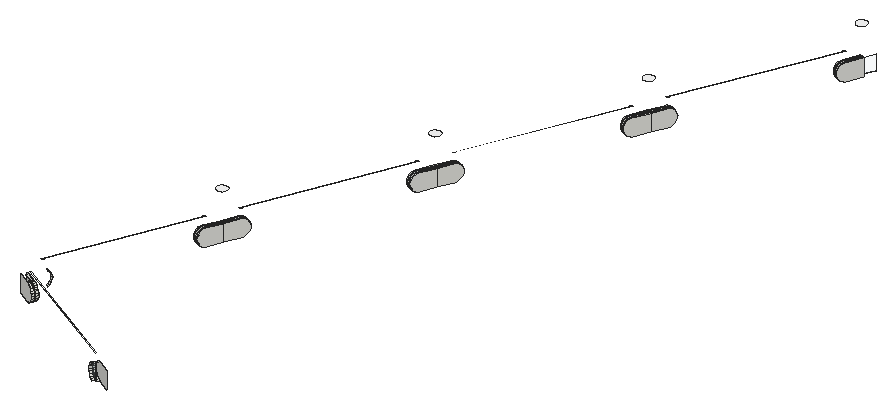
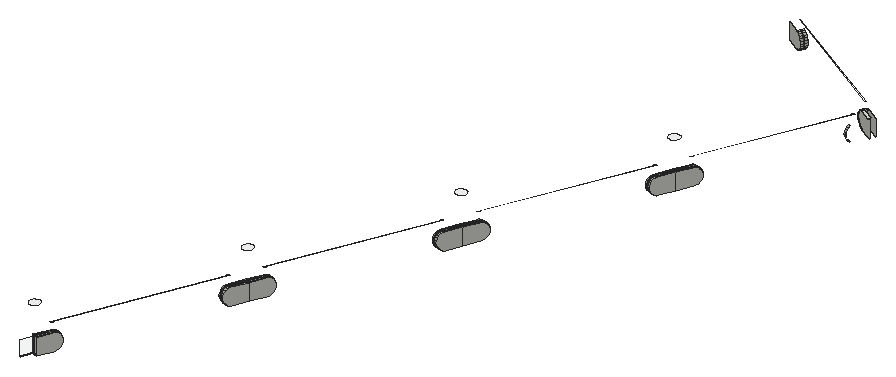
# SketchUp Ruby script. Lengths in inches.
U = 1.inch
M = Sketchup.active_model
def pt(a) = Geom::Point3d.new(a.map { |v| v * U })
def face(e, loops, mat)
  f = e.add_face(loops[0].map { |a| pt(a) })
  loops[1..].each { |l| e.add_face(l.map { |a| pt(a) }).erase! }
  f.material = f.back_material = mat if mat
  f
end
# faces: each face lists its corners as indices into pts; further lists are holes
def faces(e, pts, list, mat = nil) = list.each { |f| face(e, (f[0].is_a?(Array) ? f : [f]).map { |l| l.map { |i| pts[i] } }, mat) }
# xy, xz, yz: faces in a plane at the given z, y or x. An outline is a flat list of corners, or four numbers for a rectangle; further outlines are holes
def ring(l) = l.size == 4 ? [[l[0], l[1]], [l[2], l[1]], [l[2], l[3]], [l[0], l[3]]] : l.each_slice(2).to_a
def flat(e, list, mat, &to3) = list.each { |f| face(e, (f[0].is_a?(Array) ? f : [f]).map { |l| ring(l).map { |u, v| to3.(u, v) } }, mat) }
def xy(e, z, list, mat = nil) = flat(e, list, mat) { |x, y| [x, y, z] }
def xz(e, y, list, mat = nil) = flat(e, list, mat) { |x, z| [x, y, z] }
def yz(e, x, list, mat = nil) = flat(e, list, mat) { |y, z| [x, y, z] }
def lines(e, pts, list) = list.each { |a, b| e.add_line(pt(pts[a]), pt(pts[b])) }
# prism: a flat outline (further loops are holes) pulled along v
def prism(e, loops, v, mat = nil)
  f = face(e, loops, mat); d = Geom::Vector3d.new(v.map { |x| x * U })
  f.pushpull(f.normal.samedirection?(d) ? d.length : -d.length)
end
def box(e, o, s, mat = nil) = prism(e, [[o, [o[0] + s[0], o[1], o[2]], [o[0] + s[0], o[1] + s[1], o[2]], [o[0], o[1] + s[1], o[2]]]], [0, 0, s[2]], mat)
def at(x, y, z, deg = 0) = Geom::Transformation.translation(pt([x, y, z])) * Geom::Transformation.rotation(ORIGIN, Z_AXIS, deg.degrees)
def axes(o, x, y, z) = Geom::Transformation.new([*x, 0, *y, 0, *z, 0, *pt(o).to_a, 1])
def part(name) = M.definitions.add(name)
# library, detail: a bought-in or finely detailed component or shape, given as its bounding box
def library(name, o, s) = part(name).tap { |d| box(d.entities, o, s) }
def detail(e, o, s) = box(e.add_group.entities, o, s)
def put(e, d, t, mat = nil) = e.add_instance(d, t).tap { |i| i.material = mat if mat }
def group(e, t, mat = nil) = e.add_group.tap { |g| g.transformation = t; g.material = mat if mat }.entities
root = M.entities
M.materials.add("Glass_Safety_01").color = [204, 235, 244]
M.materials["Glass_Safety_01"].alpha = 0.1
M.materials.add("[Color_000]").color = [255, 255, 255]
xy(root,351.28,[[970.32,886.89,970.06,887,970.13,887.16,970.85,888.81,971.1,888.7],[969.88,887.08,969.63,887.1875,970.42,888.99,970.67,888.88,969.95,887.24],[971.1,888.7,970.85,888.81,971.64,890.61,971.89,890.5],[970.67,888.88,970.42,888.99,971.2,890.8,971.46,890.6875],[979.95,909,979.69,909.11,979.76,909.25,980.48,910.91,980.73,910.8],
  [979.51,909.1875,979.26,909.3,980.05,911.1,980.3,910.99,979.58,909.33],[980.73,910.8,980.48,910.91,981.27,912.72,981.52,912.61],[980.3,910.99,980.05,911.1,980.83,912.91,981.08,912.8],[989.59,931.14,989.34,931.25,989.4,931.39,990.12,933.05,990.375,932.94],[989.16,931.33,988.9,931.4375,989.6875,933.24,989.94,933.13,989.22,931.47],
  [990.375,932.94,990.12,933.05,990.91,934.86,991.16,934.75],[989.94,933.13,989.6875,933.24,990.47,935.05,990.73,934.9375],[999.21,953.22,998.95,953.33,999.02,953.48,999.74,955.13,999.99,955.02],[998.77,953.41,998.52,953.52,999.31,955.32,999.56,955.21,998.84,953.56]])
xy(root,351.36,[[970.22,887.36,970.04,887.44,970.67,888.88,970.85,888.81],[970.85,888.81,970.67,888.88,971.3,890.33,971.48,890.25],[979.85,909.47,979.67,909.55,980.3,910.99,980.48,910.91],[980.48,910.91,980.3,910.99,980.93,912.43,981.11,912.36],[989.49,931.61,989.3125,931.6875,989.94,933.13,990.12,933.05],
  [990.12,933.05,989.94,933.13,990.57,934.57,990.75,934.5],[999.11,953.69,998.93,953.77,999.56,955.21,999.74,955.13],[999.74,955.13,999.56,955.21,1000.1875,956.66,1000.37,956.58]],"Glass_Safety_01")
xy(root,353.33,[[970.22,887.36,970.85,888.81,970.67,888.88,970.04,887.44],[970.85,888.81,971.48,890.25,971.3,890.33,970.67,888.88],[979.85,909.47,980.48,910.91,980.3,910.99,979.67,909.55],[980.48,910.91,981.11,912.36,980.93,912.43,980.3,910.99],[989.49,931.61,990.12,933.05,989.94,933.13,989.3125,931.6875],
  [990.12,933.05,990.75,934.5,990.57,934.57,989.94,933.13],[999.11,953.69,999.74,955.13,999.56,955.21,998.93,953.77]],"Glass_Safety_01")
xy(root,353.41,[[963.5625,867.39,963.7,867.63,962.28,868.4375,962.17,868.18,963.41,867.48],[970.32,886.89,971.1,888.7,970.85,888.81,970.13,887.16,970.06,887],[969.88,887.08,969.95,887.24,970.67,888.88,970.42,888.99,969.63,887.1875],[971.1,888.7,971.89,890.5,971.64,890.61,970.85,888.81],[970.67,888.88,971.46,890.6875,971.2,890.8,970.42,888.99],
  [979.95,909,980.73,910.8,980.48,910.91,979.76,909.25,979.69,909.11],[979.51,909.1875,979.58,909.33,980.3,910.99,980.05,911.1,979.26,909.3],[980.73,910.8,981.52,912.61,981.27,912.72,980.48,910.91],[980.3,910.99,981.08,912.8,980.83,912.91,980.05,911.1],[989.59,931.14,990.375,932.94,990.12,933.05,989.4,931.39,989.34,931.25],
  [989.16,931.33,989.22,931.47,989.94,933.13,989.6875,933.24,988.9,931.4375],[990.375,932.94,991.16,934.75,990.91,934.86,990.12,933.05],[989.94,933.13,990.73,934.9375,990.47,935.05,989.6875,933.24],[999.21,953.22,999.99,955.02,999.74,955.13,999.02,953.48,998.95,953.33],[998.77,953.41,998.84,953.56,999.56,955.21,999.31,955.32,998.52,953.52]])
xy(root,354.51,[[978.84,858.44,978.9375,858.62,963.31,867.31],[978.9375,858.62,963.41,867.48,963.31,867.31],[962.68,870.04,969.95,887.24,962.5,870.12],[962.68,870.04,970.13,887.16,969.95,887.24],[971.64,890.61,979.58,909.33,971.46,890.6875],
  [971.64,890.61,979.76,909.25,979.58,909.33],[981.27,912.72,989.22,931.47,981.08,912.8],[981.27,912.72,989.4,931.39,989.22,931.47],[990.91,934.86,998.84,953.56,990.73,934.9375],[990.91,934.86,999.02,953.48,998.84,953.56]],"Glass_Safety_01")
xy(root,357.27,[[970.81,888.22,970.97,888.25,971.11,888.32,971.24,888.43,971.33,888.57,971.38,888.73,971.39,888.89,971.36,889.05,971.28,889.2,971.17,889.32,971.04,889.41,970.88,889.46,970.72,889.47,970.55,889.44,970.41,889.37,970.28,889.26,970.19,889.12,970.14,888.96,970.13,888.8,970.17,888.64,970.24,888.49,970.35,888.37,970.49,888.28,970.64,888.23],[980.43,910.32,980.6,910.36,980.74,910.43,980.87,910.54,980.96,910.68,981.01,910.83,981.02,911,980.98,911.16,980.91,911.3,980.8,911.43,980.66,911.52,980.51,911.57,980.34,911.58,980.18,911.55,980.04,911.47,979.91,911.36,979.82,911.23,979.77,911.07,979.76,910.91,979.79,910.75,979.87,910.6,979.98,910.48,980.11,910.39,980.27,910.33],[990.08,932.46,990.24,932.5,990.38,932.57,990.51,932.68,990.6,932.82,990.65,932.97,990.66,933.14,990.625,933.3,990.55,933.44,990.44,933.57,990.31,933.66,990.15,933.71,989.99,933.72,989.83,933.6875,989.68,933.61,989.56,933.5,989.46,933.37,989.41,933.21,989.4,933.05,989.4375,932.89,989.51,932.74,989.62,932.62,989.76,932.53,989.91,932.47],[999.69,954.54,999.85,954.58,1000,954.65,1000.125,954.76,1000.22,954.9,1000.27,955.05,1000.28,955.22,1000.24,955.38,1000.17,955.53,1000.0625,955.65,999.92,955.74,999.77,955.79,999.6,955.8,999.44,955.77,999.3,955.69,999.17,955.59,999.08,955.45,999.03,955.29,999.02,955.13,999.05,954.97,999.13,954.82,999.24,954.7,999.375,954.61,999.53,954.55]],"[Color_000]")
p = [[980.72,857.91,353.41],[980.78,857.88,353.41],[980.78,857.88,351.28],[980.72,857.91,351.28],[979.07,858.85,351.28],[978.83,858.99,351.32],
  [978.61,859.12,351.43],[978.42,859.23,351.59],[978.27,859.3125,351.8125],[978.18,859.36,352.07],[978.15,859.38,352.35],[978.18,859.36,352.62],
  [978.27,859.3125,352.88],[978.42,859.23,353.1],[978.61,859.12,353.27],[978.83,858.99,353.37],[979.07,858.85,353.41],[978.375,858.71,351.43],
  [978.6,858.58,351.32],[978.46,858.34,351.32],[978.24,858.47,351.43],[978.84,858.44,351.28],[978.84,858.44,353.41],[978.6,858.58,353.37],
  [978.375,858.71,353.27],[978.1875,858.82,353.1],[978.04,858.9,352.88],[977.95,858.95,352.62],[977.92,858.97,352.35],[977.95,858.95,352.07],
  [978.04,858.9,351.8125],[978.1875,858.82,351.59],[978.9375,858.62,353.41],[978.9375,858.62,351.28],[978.7,858.75,351.32],[978.47,858.88,351.43],
  [978.28,858.99,351.59],[978.14,859.07,351.8125],[978.04,859.125,352.07],[978.01,859.14,352.35],[978.04,859.125,352.62],[978.14,859.07,352.88],
  [978.28,858.99,353.1],[978.47,858.88,353.27],[978.7,858.75,353.37],[963.33,866.98,353.41],[961.62,867.95,353.41],[961.62,867.95,351.28],
  [963.33,866.98,351.28],[963.57,866.84,351.32],[963.79,866.71,351.43],[963.98,866.61,351.59],[964.13,866.52,351.8125],[964.22,866.47,352.07],
  [964.25,866.45,352.35],[964.22,866.47,352.62],[964.13,866.52,352.88],[963.98,866.61,353.1],[963.79,866.71,353.27],[963.57,866.84,353.37],
  [963.46,867.22,351.28],[963.31,867.31,351.28],[963.31,867.31,353.41],[963.46,867.22,353.41],[963.7,867.08,353.37],[963.93,866.95,353.27],
  [964.12,866.84,353.1],[964.26,866.76,352.88],[964.36,866.71,352.62],[964.39,866.69,352.35],[964.36,866.71,352.07],[964.26,866.76,351.8125],
  [964.12,866.84,351.59],[963.93,866.95,351.43],[963.7,867.08,351.32],[963.5625,867.39,353.41],[963.41,867.48,353.41],[963.41,867.48,351.28],
  [963.5625,867.39,351.28],[963.8,867.25,351.32],[964.02,867.125,351.43],[964.21,867.02,351.59],[964.36,866.93,351.8125],[964.45,866.88,352.07],
  [964.49,866.86,352.35],[964.45,866.88,352.62],[964.36,866.93,352.88],[964.21,867.02,353.1],[964.02,867.125,353.27],[963.8,867.25,353.37],
  [961.99,868.6,353.41],[962.04,868.57,353.41],[962.28,868.4375,353.41],[963.7,867.63,353.41],[963.9375,867.49,353.37],[964.16,867.36,353.27],
  [964.35,867.25,353.1],[964.5,867.17,352.88],[964.59,867.12,352.62],[964.62,867.1,352.35],[964.59,867.12,352.07],[964.5,867.17,351.8125],
  [964.35,867.25,351.59],[964.16,867.36,351.43],[963.9375,867.49,351.32],[963.7,867.63,351.28],[962.28,868.4375,351.28],[962.04,868.57,351.28],
  [961.99,868.6,351.28],[971.1,888.7,353.41],[970.32,886.89,353.41],[970.21,886.64,353.37],[970.11,886.4,353.27],[970.02,886.2,353.1],
  [969.95,886.05,352.88],[969.91,885.95,352.62],[969.89,885.92,352.35],[969.91,885.95,352.07],[969.95,886.05,351.8125],[970.02,886.2,351.59],
  [970.11,886.4,351.43],[970.21,886.64,351.32],[970.32,886.89,351.28],[971.1,888.7,351.28],[970.06,887,353.41],[970.13,887.16,353.41],
  [970.13,887.16,351.28],[970.06,887,351.28],[969.96,886.75,351.32],[969.85,886.51,351.43],[969.76,886.3125,351.59],[969.7,886.16,351.8125],
  [969.65,886.06,352.07],[969.64,886.03,352.35],[969.65,886.06,352.62],[969.7,886.16,352.88],[969.76,886.3125,353.1],[969.85,886.51,353.27],
  [969.96,886.75,353.37],[969.88,887.08,351.28],[969.95,887.24,351.28],[969.95,887.24,353.41],[969.88,887.08,353.41],[969.77,886.83,353.37],
  [969.67,886.59,353.27],[969.58,886.39,353.1],[969.52,886.24,352.88],[969.47,886.14,352.62],[969.46,886.1,352.35],[969.47,886.14,352.07],
  [969.52,886.24,351.8125],[969.58,886.39,351.59],[969.67,886.59,351.43],[969.77,886.83,351.32],[969.63,887.1875,353.41],[970.42,888.99,353.41],
  [970.42,888.99,351.28],[969.63,887.1875,351.28],[969.52,886.9375,351.32],[969.42,886.7,351.43],[969.33,886.5,351.59],[969.26,886.35,351.8125],
  [969.22,886.25,352.07],[969.21,886.21,352.35],[969.22,886.25,352.62],[969.26,886.35,352.88],[969.33,886.5,353.1],[969.42,886.7,353.27],
  [969.52,886.9375,353.37],[970.67,888.88,353.41],[970.67,888.88,351.28],[970.67,888.88,351.36],[970.04,887.44,351.36],[970.04,887.44,353.33],
  [970.67,888.88,353.33],[970.85,888.81,351.28],[970.85,888.81,353.41],[970.85,888.81,353.33],[970.22,887.36,353.33],[970.22,887.36,351.36],
  [970.85,888.81,351.36],[971.89,890.5,353.41],[971.89,890.5,351.28],[972,890.75,351.32],[972.1,890.99,351.43],[972.19,891.1875,351.59],
  [972.26,891.34,351.8125],[972.3,891.44,352.07],[972.3125,891.47,352.35],[972.3,891.44,352.62],[972.26,891.34,352.88],[972.19,891.1875,353.1],
  [972.1,890.99,353.27],[972,890.75,353.37],[971.64,890.61,353.41],[971.64,890.61,351.28],[971.48,890.25,351.36],[971.48,890.25,353.33],
  [971.46,890.6875,351.28],[971.46,890.6875,353.41],[971.3,890.33,353.33],[971.3,890.33,351.36],[971.2,890.8,353.41],[971.3125,891.05,353.37],
  [971.42,891.29,353.27],[971.5,891.49,353.1],[971.57,891.64,352.88],[971.61,891.74,352.62],[971.63,891.77,352.35],[971.61,891.74,352.07],
  [971.57,891.64,351.8125],[971.5,891.49,351.59],[971.42,891.29,351.43],[971.3125,891.05,351.32],[971.2,890.8,351.28],[971.75,890.86,351.32],
  [971.85,891.1,351.43],[971.9375,891.3,351.59],[972,891.45,351.8125],[972.05,891.55,352.07],[972.0625,891.58,352.35],[972.05,891.55,352.62],
  [972,891.45,352.88],[971.9375,891.3,353.1],[971.85,891.1,353.27],[971.75,890.86,353.37],[971.57,890.94,351.32],[971.57,890.94,353.37],
  [971.67,891.18,353.27],[971.76,891.38,353.1],[971.82,891.53,352.88],[971.87,891.63,352.62],[971.88,891.66,352.35],[971.87,891.63,352.07],
  [971.82,891.53,351.8125],[971.76,891.38,351.59],[971.67,891.18,351.43],[980.73,910.8,353.41],[979.95,909,353.41],[979.84,908.75,353.37],
  [979.73,908.51,353.27],[979.65,908.31,353.1],[979.58,908.15,352.88],[979.54,908.06,352.62],[979.52,908.02,352.35],[979.54,908.06,352.07],
  [979.58,908.15,351.8125],[979.65,908.31,351.59],[979.73,908.51,351.43],[979.84,908.75,351.32],[979.95,909,351.28],[980.73,910.8,351.28],
  [979.69,909.11,353.41],[979.76,909.25,353.41],[979.76,909.25,351.28],[979.69,909.11,351.28],[979.58,908.86,351.32],[979.48,908.62,351.43],
  [979.39,908.42,351.59],[979.33,908.26,351.8125],[979.28,908.17,352.07],[979.27,908.13,352.35],[979.28,908.17,352.62],[979.33,908.26,352.88],
  [979.39,908.42,353.1],[979.48,908.62,353.27],[979.58,908.86,353.37],[979.51,909.1875,351.28],[979.58,909.33,351.28],[979.58,909.33,353.41],
  [979.51,909.1875,353.41],[979.4,908.93,353.37],[979.3,908.7,353.27],[979.21,908.5,353.1],[979.15,908.34,352.88],[979.1,908.24,352.62],
  [979.09,908.21,352.35],[979.1,908.24,352.07],[979.15,908.34,351.8125],[979.21,908.5,351.59],[979.3,908.7,351.43],[979.4,908.93,351.32],
  [979.26,909.3,353.41],[980.05,911.1,353.41],[980.05,911.1,351.28],[979.26,909.3,351.28],[979.15,909.04,351.32],[979.05,908.81,351.43],
  [978.96,908.61,351.59],[978.89,908.45,351.8125],[978.85,908.35,352.07],[978.84,908.32,352.35],[978.85,908.35,352.62],[978.89,908.45,352.88],
  [978.96,908.61,353.1],[979.05,908.81,353.27],[979.15,909.04,353.37],[980.3,910.99,353.41],[980.3,910.99,351.28],[980.3,910.99,351.36],
  [979.67,909.55,351.36],[979.67,909.55,353.33],[980.3,910.99,353.33],[980.48,910.91,351.28],[980.48,910.91,353.41],[980.48,910.91,353.33],
  [979.85,909.47,353.33],[979.85,909.47,351.36],[980.48,910.91,351.36],[981.52,912.61,353.41],[981.52,912.61,351.28],[981.63,912.86,351.32],
  [981.73,913.09,351.43],[981.82,913.3,351.59],[981.89,913.45,351.8125],[981.93,913.55,352.07],[981.94,913.58,352.35],[981.93,913.55,352.62],
  [981.89,913.45,352.88],[981.82,913.3,353.1],[981.73,913.09,353.27],[981.63,912.86,353.37],[981.27,912.72,353.41],[981.27,912.72,351.28],
  [981.11,912.36,351.36],[981.11,912.36,353.33],[981.08,912.8,351.28],[981.08,912.8,353.41],[980.93,912.43,353.33],[980.93,912.43,351.36],
  [980.83,912.91,353.41],[980.94,913.16,353.37],[981.04,913.39,353.27],[981.13,913.59,353.1],[981.2,913.75,352.88],[981.24,913.85,352.62],
  [981.26,913.88,352.35],[981.24,913.85,352.07],[981.2,913.75,351.8125],[981.13,913.59,351.59],[981.04,913.39,351.43],[980.94,913.16,351.32],
  [980.83,912.91,351.28],[981.375,912.97,351.32],[981.48,913.2,351.43],[981.57,913.41,351.59],[981.63,913.5625,351.8125],[981.68,913.66,352.07],
  [981.69,913.69,352.35],[981.68,913.66,352.62],[981.63,913.5625,352.88],[981.57,913.41,353.1],[981.48,913.2,353.27],[981.375,912.97,353.37],
  [981.19,913.05,351.32],[981.19,913.05,353.37],[981.3,913.28,353.27],[981.38,913.48,353.1],[981.45,913.64,352.88],[981.49,913.74,352.62],
  [981.51,913.77,352.35],[981.49,913.74,352.07],[981.45,913.64,351.8125],[981.38,913.48,351.59],[981.3,913.28,351.43],[990.375,932.94,353.41],
  [989.59,931.14,353.41],[989.48,930.89,353.37],[989.375,930.65,353.27],[989.29,930.45,353.1],[989.22,930.29,352.88],[989.18,930.2,352.62],
  [989.16,930.16,352.35],[989.18,930.2,352.07],[989.22,930.29,351.8125],[989.29,930.45,351.59],[989.375,930.65,351.43],[989.48,930.89,351.32],
  [989.59,931.14,351.28],[990.375,932.94,351.28],[989.34,931.25,353.41],[989.4,931.39,353.41],[989.4,931.39,351.28],[989.34,931.25,351.28],
  [989.23,931,351.32],[989.125,930.76,351.43],[989.04,930.56,351.59],[988.97,930.4,351.8125],[988.93,930.31,352.07],[988.91,930.27,352.35],
  [988.93,930.31,352.62],[988.97,930.4,352.88],[989.04,930.56,353.1],[989.125,930.76,353.27],[989.23,931,353.37],[989.16,931.33,351.28],
  [989.22,931.47,351.28],[989.22,931.47,353.41],[989.16,931.33,353.41],[989.05,931.07,353.37],[988.94,930.84,353.27],[988.86,930.64,353.1],
  [988.79,930.48,352.88],[988.75,930.38,352.62],[988.73,930.35,352.35],[988.75,930.38,352.07],[988.79,930.48,351.8125],[988.86,930.64,351.59],
  [988.94,930.84,351.43],[989.05,931.07,351.32],[988.9,931.4375,353.41],[989.6875,933.24,353.41],[989.6875,933.24,351.28],[988.9,931.4375,351.28],
  [988.79,931.18,351.32],[988.69,930.95,351.43],[988.6,930.75,351.59],[988.54,930.59,351.8125],[988.49,930.5,352.07],[988.48,930.46,352.35],
  [988.49,930.5,352.62],[988.54,930.59,352.88],[988.6,930.75,353.1],[988.69,930.95,353.27],[988.79,931.18,353.37],[990.12,933.05,351.28],
  [990.12,933.05,353.41],[990.12,933.05,353.33],[989.49,931.61,353.33],[989.49,931.61,351.36],[990.12,933.05,351.36],[989.94,933.13,353.41],
  [989.94,933.13,351.28],[989.94,933.13,351.36],[989.3125,931.6875,351.36],[989.3125,931.6875,353.33],[989.94,933.13,353.33],[991.16,934.75,353.41],
  [991.16,934.75,351.28],[991.27,935,351.32],[991.37,935.23,351.43],[991.46,935.4375,351.59],[991.53,935.59,351.8125],[991.57,935.6875,352.07],
  [991.59,935.72,352.35],[991.57,935.6875,352.62],[991.53,935.59,352.88],[991.46,935.4375,353.1],[991.37,935.23,353.27],[991.27,935,353.37],
  [990.73,934.9375,351.28],[990.73,934.9375,353.41],[990.57,934.57,353.33],[990.57,934.57,351.36],[990.91,934.86,353.41],[990.91,934.86,351.28],
  [990.75,934.5,351.36],[990.75,934.5,353.33],[990.47,935.05,353.41],[990.58,935.3,353.37],[990.6875,935.53,353.27],[990.77,935.74,353.1],
  [990.84,935.89,352.88],[990.88,935.99,352.62],[990.9,936.02,352.35],[990.88,935.99,352.07],[990.84,935.89,351.8125],[990.77,935.74,351.59],
  [990.6875,935.53,351.43],[990.58,935.3,351.32],[990.47,935.05,351.28],[991.02,935.11,351.32],[990.84,935.1875,351.32],[990.84,935.1875,353.37],
  [990.94,935.42,353.27],[991.03,935.625,353.1],[991.1,935.78,352.88],[991.14,935.88,352.62],[991.15,935.91,352.35],[991.14,935.88,352.07],
  [991.1,935.78,351.8125],[991.03,935.625,351.59],[990.94,935.42,351.43],[991.12,935.34,351.43],[991.21,935.55,351.59],[991.28,935.7,351.8125],
  [991.32,935.8,352.07],[991.33,935.83,352.35],[991.32,935.8,352.62],[991.28,935.7,352.88],[991.21,935.55,353.1],[991.12,935.34,353.27],
  [991.02,935.11,353.37],[999.99,955.02,353.41],[999.21,953.22,353.41],[999.1,952.97,353.37],[998.99,952.73,353.27],[998.91,952.53,353.1],
  [998.84,952.375,352.88],[998.8,952.28,352.62],[998.78,952.24,352.35],[998.8,952.28,352.07],[998.84,952.375,351.8125],[998.91,952.53,351.59],
  [998.99,952.73,351.43],[999.1,952.97,351.32],[999.21,953.22,351.28],[999.99,955.02,351.28],[998.77,953.41,351.28],[998.84,953.56,351.28],
  [998.84,953.56,353.41],[998.77,953.41,353.41],[998.66,953.16,353.37],[998.56,952.92,353.27],[998.47,952.72,353.1],[998.4,952.5625,352.88],
  [998.36,952.47,352.62],[998.35,952.43,352.35],[998.36,952.47,352.07],[998.4,952.5625,351.8125],[998.47,952.72,351.59],[998.56,952.92,351.43],
  [998.66,953.16,351.32],[998.95,953.33,353.41],[999.02,953.48,353.41],[999.02,953.48,351.28],[998.95,953.33,351.28],[998.84,953.08,351.32],
  [998.74,952.84,351.43],[998.65,952.64,351.59],[998.59,952.49,351.8125],[998.54,952.39,352.07],[998.53,952.35,352.35],[998.54,952.39,352.62],
  [998.59,952.49,352.88],[998.65,952.64,353.1],[998.74,952.84,353.27],[998.84,953.08,353.37],[998.52,953.52,353.41],[999.31,955.32,353.41],
  [999.31,955.32,351.28],[998.52,953.52,351.28],[998.41,953.27,351.32],[998.31,953.03,351.43],[998.22,952.83,351.59],[998.15,952.67,351.8125],
  [998.11,952.58,352.07],[998.1,952.54,352.35],[998.11,952.58,352.62],[998.15,952.67,352.88],[998.22,952.83,353.1],[998.31,953.03,353.27],
  [998.41,953.27,353.37],[999.74,955.13,351.28],[999.74,955.13,353.41],[999.74,955.13,353.33],[999.11,953.69,353.33],[999.11,953.69,351.36],
  [999.74,955.13,351.36],[999.56,955.21,353.41],[999.56,955.21,351.28],[999.56,955.21,351.36],[998.93,953.77,351.36],[998.93,953.77,353.33],
  [999.56,955.21,353.33],[978.05,858.58,351.59],[963.12,867.41,353.33],[963.12,867.41,351.36],[963.22,867.58,351.36],[963.22,867.58,353.33],
  [962.89,870.53,351.43],[962.98,870.73,351.59],[963.23,870.62,351.59],[963.14,870.42,351.43],[1000.37,956.58,353.33],[1000.37,956.58,351.36],
  [977.9,858.66,351.8125],[963.05,870.89,351.8125],[963.3,870.78,351.8125],[977.81,858.71,352.07],[963.09,870.99,352.07],[963.34,870.875,352.07],
  [977.78,858.73,352.35],[963.1,871.02,352.35],[963.36,870.91,352.35],[977.81,858.71,352.62],[963.09,870.99,352.62],[963.34,870.875,352.62],
  [977.9,858.66,352.88],[963.05,870.89,352.88],[963.3,870.78,352.88],[978.05,858.58,353.1],[962.98,870.73,353.1],[963.23,870.62,353.1],
  [978.24,858.47,353.27],[962.89,870.53,353.27],[963.14,870.42,353.27],[978.46,858.34,353.37],[978.7,858.21,353.41]]
faces(root,p,[[0,1,2,3,4,5,6,7,8,9,10,11,12,13,14,15,16],[17,18,19,20],[33,34,5,4],[34,35,6,5],[45,46,47,48,49,50,51,52,53,54,55,56,57,58,59],[60,61,62,63,64,65,66,67,68,69,70,71,72,73,74],[74,73,50,49],[60,74,49,48],
  [75,76,77,78,79,80,81,82,83,84,85,86,87,88,89],[90,91,92,93,94,95,96,97,98,99,100,101,102,103,104,105,106,107,108],[80,79,104,103],[79,78,105,104],[109,110,111,112,113,114,115,116,117,118,119,120,121,122,123],[124,125,126,127,128,129,130,131,132,133,134,135,136,137,138],[139,140,141,142,143,144,145,146,147,148,149,150,151,152,153],[154,155,156,157,158,159,160,161,162,163,164,165,166,167,168],
  [129,128,121,120],[153,152,159,158],[128,127,122,121],[139,153,158,157],[169,141,140,170,171,172,173,174],[175,126,125,176,177,178,179,180],[175,180,177,176,109,123],[181,109,123,182,183,184,185,186,187,188,189,190,191,192,193],
  [176,194,195,175,180,196,197,177],[171,170,156,155,169,174],[170,198,199,169,174,200,201,171],[155,202,203,204,205,206,207,208,209,210,211,212,213,214,156],[195,215,183,182],[226,198,214,213],[215,216,184,183],[236,226,213,212],
  [237,238,239,240,241,242,243,244,245,246,247,248,249,250,251],[252,253,254,255,256,257,258,259,260,261,262,263,264,265,266],[267,268,269,270,271,272,273,274,275,276,277,278,279,280,281],[282,283,284,285,286,287,288,289,290,291,292,293,294,295,296],[257,256,249,248],[281,280,287,286],[256,255,250,249],[267,281,286,285],
  [297,269,268,298,299,300,301,302],[303,254,253,304,305,306,307,308],[303,308,305,304,237,251],[309,237,251,310,311,312,313,314,315,316,317,318,319,320,321],[304,322,323,303,308,324,325,305],[299,298,284,283,297,302],[298,326,327,297,302,328,329,299],[283,330,331,332,333,334,335,336,337,338,339,340,341,342,284],
  [323,343,311,310],[354,326,342,341],[343,344,312,311],[364,354,341,340],[365,366,367,368,369,370,371,372,373,374,375,376,377,378,379],[380,381,382,383,384,385,386,387,388,389,390,391,392,393,394],[395,396,397,398,399,400,401,402,403,404,405,406,407,408,409],[410,411,412,413,414,415,416,417,418,419,420,421,422,423,424],
  [385,384,377,376],[409,408,415,414],[384,383,378,377],[395,409,414,413],[425,382,381,426,427,428,429,430],[431,397,396,432,433,434,435,436],[425,430,427,426,365,379],[437,365,379,438,439,440,441,442,443,444,445,446,447,448,449],
  [433,432,412,411,431,436],[432,450,451,431,436,452,453,433],[426,454,455,425,430,456,457,427],[411,458,459,460,461,462,463,464,465,466,467,468,469,470,412],[455,471,439,438],[472,450,470,469],[471,483,440,439],[482,472,469,468],
  [493,494,495,496,497,498,499,500,501,502,503,504,505,506,507],[508,509,510,511,512,513,514,515,516,517,518,519,520,521,522],[523,524,525,526,527,528,529,530,531,532,533,534,535,536,537],[538,539,540,541,542,543,544,545,546,547,548,549,550,551,552],[528,527,505,504],[522,521,543,542],[527,526,506,505],[508,522,542,541],
  [553,525,524,554,555,556,557,558],[559,510,509,560,561,562,563,564],[553,558,555,554,493,507],[561,560,540,539,559,564],[31,17,20,565],[35,36,7,6],[73,72,51,50],[81,80,103,102],
  [570,571,572,573],[130,129,120,119],[152,151,160,159],[216,217,185,184],[235,236,212,211],[258,257,248,247],[280,279,288,287],[344,345,313,312],
  [363,364,340,339],[386,385,376,375],[408,407,416,415],[483,484,441,440],[481,482,468,467],[529,528,504,503],[521,520,544,543],[30,31,565,576],
  [36,37,8,7],[72,71,52,51],[82,81,102,101],[571,577,578,572],[131,130,119,118],[151,150,161,160],[217,218,186,185],[234,235,211,210],
  [259,258,247,246],[279,278,289,288],[345,346,314,313],[362,363,339,338],[387,386,375,374],[407,406,417,416],[484,485,442,441],[480,481,467,466],
  [530,529,503,502],[520,519,545,544],[29,30,576,579],[37,38,9,8],[71,70,53,52],[83,82,101,100],[577,580,581,578],[132,131,118,117],
  [150,149,162,161],[218,219,187,186],[233,234,210,209],[260,259,246,245],[278,277,290,289],[346,347,315,314],[361,362,338,337],[388,387,374,373],
  [406,405,418,417],[485,486,443,442],[479,480,466,465],[531,530,502,501],[519,518,546,545],[28,29,579,582],[38,39,10,9],[70,69,54,53],
  [84,83,100,99],[580,583,584,581],[133,132,117,116],[149,148,163,162],[219,220,188,187],[232,233,209,208],[261,260,245,244],[277,276,291,290],
  [347,348,316,315],[360,361,337,336],[389,388,373,372],[405,404,419,418],[486,487,444,443],[478,479,465,464],[532,531,501,500],[518,517,547,546],
  [27,28,582,585],[39,40,11,10],[69,68,55,54],[85,84,99,98],[583,586,587,584],[134,133,116,115],[148,147,164,163],[220,221,189,188],
  [231,232,208,207],[262,261,244,243],[276,275,292,291],[348,349,317,316],[359,360,336,335],[390,389,372,371],[404,403,420,419],[487,488,445,444],
  [477,478,464,463],[533,532,500,499],[517,516,548,547],[26,27,585,588],[40,41,12,11],[68,67,56,55],[86,85,98,97],[586,589,590,587],
  [135,134,115,114],[147,146,165,164],[221,222,190,189],[230,231,207,206],[263,262,243,242],[275,274,293,292],[349,350,318,317],[358,359,335,334],
  [391,390,371,370],[403,402,421,420],[488,489,446,445],[476,477,463,462],[534,533,499,498],[516,515,549,548],[25,26,588,591],[41,42,13,12],
  [67,66,57,56],[87,86,97,96],[589,592,593,590],[136,135,114,113],[146,145,166,165],[222,223,191,190],[229,230,206,205],[264,263,242,241],
  [274,273,294,293],[350,351,319,318],[357,358,334,333],[392,391,370,369],[402,401,422,421],[489,490,447,446],[475,476,462,461],[535,534,498,497],
  [515,514,550,549],[24,25,591,594],[42,43,14,13],[66,65,58,57],[88,87,96,95],[592,595,596,593],[137,136,113,112],[145,144,167,166],
  [223,224,192,191],[228,229,205,204],[265,264,241,240],[273,272,295,294],[351,352,320,319],[356,357,333,332],[393,392,369,368],[401,400,423,422],
  [490,491,448,447],[474,475,461,460],[536,535,497,496],[514,513,551,550],[23,24,594,597],[43,44,15,14],[65,64,59,58],[89,88,95,94],
  [138,137,112,111],[144,143,168,167],[224,225,193,192],[227,228,204,203],[266,265,240,239],[272,271,296,295],[352,353,321,320],[355,356,332,331],
  [394,393,368,367],[400,399,424,423],[491,492,449,448],[473,474,460,459],[537,536,496,495],[513,512,552,551],[22,23,597,598],[44,32,16,15],
  [64,63,45,59],[75,89,94,93],[124,138,111,110],[143,142,154,168],[225,194,181,193],[199,227,203,202],[252,266,239,238],[271,270,282,296],
  [353,322,309,321],[327,355,331,330],[380,394,367,366],[399,398,410,424],[492,454,437,449],[451,473,459,458],[523,537,495,494],[512,511,538,552]])
faces(root,p,[[21,22,23,24,25,26,27,28,29,30,31,17,18],[32,33,34,35,36,37,38,39,40,41,42,43,44],[194,195,215,216,217,218,219,220,221,222,223,224,225],[198,199,227,228,229,230,231,232,233,234,235,236,226],[322,323,343,344,345,346,347,348,349,350,351,352,353],[326,327,355,356,357,358,359,360,361,362,363,364,354],[450,451,473,474,475,476,477,478,479,480,481,482,472],[454,455,471,483,484,485,486,487,488,489,490,491,492],
  [566,567,568,569],[173,172,179,178],[174,173,172,171],[178,177,180,179],[174,177,180,171],[177,197,196,180],[200,174,171,201],[197,196,201,200],
  [301,300,307,306],[302,301,300,299],[306,305,308,307],[302,305,308,299],[305,325,324,308],[328,302,299,329],[325,324,329,328],[435,434,429,428],
  [428,427,430,429],[436,435,434,433],[436,427,430,433],[452,436,433,453],[427,457,456,430],[457,456,453,452],[563,562,557,556],[556,555,558,557],
  [564,563,562,561],[564,555,558,561],[555,574,575,558]],"Glass_Safety_01")
